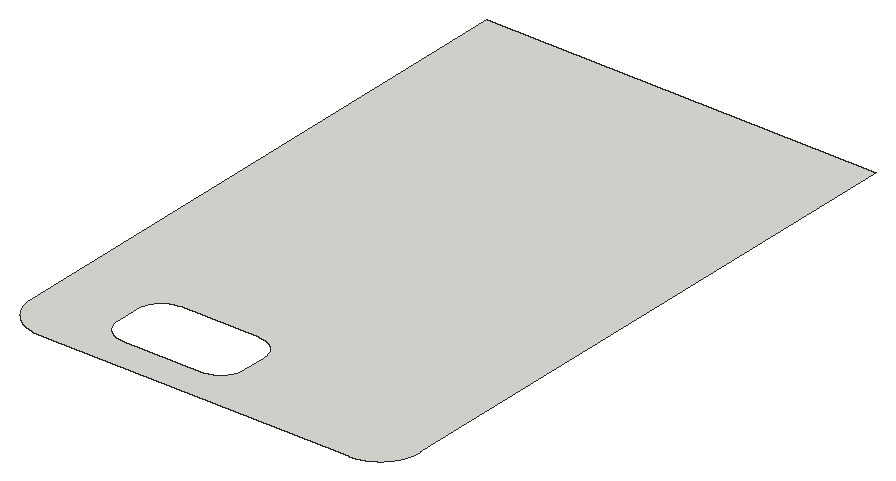
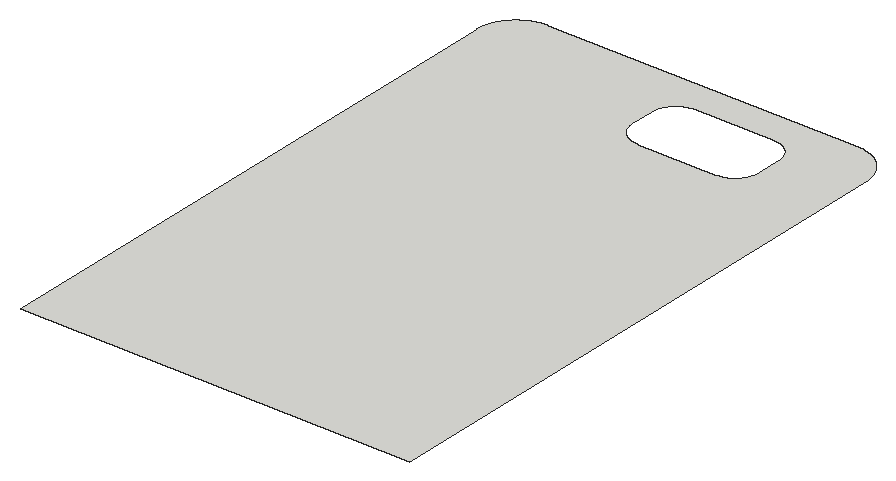
# SketchUp Ruby script. Lengths in inches.
U = 1.inch
M = Sketchup.active_model
def pt(a) = Geom::Point3d.new(a.map { |v| v * U })
def face(e, loops, mat)
  f = e.add_face(loops[0].map { |a| pt(a) })
  loops[1..].each { |l| e.add_face(l.map { |a| pt(a) }).erase! }
  f.material = f.back_material = mat if mat
  f
end
# faces: each face lists its corners as indices into pts; further lists are holes
def faces(e, pts, list, mat = nil) = list.each { |f| face(e, (f[0].is_a?(Array) ? f : [f]).map { |l| l.map { |i| pts[i] } }, mat) }
# xy, xz, yz: faces in a plane at the given z, y or x. An outline is a flat list of corners, or four numbers for a rectangle; further outlines are holes
def ring(l) = l.size == 4 ? [[l[0], l[1]], [l[2], l[1]], [l[2], l[3]], [l[0], l[3]]] : l.each_slice(2).to_a
def flat(e, list, mat, &to3) = list.each { |f| face(e, (f[0].is_a?(Array) ? f : [f]).map { |l| ring(l).map { |u, v| to3.(u, v) } }, mat) }
def xy(e, z, list, mat = nil) = flat(e, list, mat) { |x, y| [x, y, z] }
def xz(e, y, list, mat = nil) = flat(e, list, mat) { |x, z| [x, y, z] }
def yz(e, x, list, mat = nil) = flat(e, list, mat) { |y, z| [x, y, z] }
def lines(e, pts, list) = list.each { |a, b| e.add_line(pt(pts[a]), pt(pts[b])) }
# prism: a flat outline (further loops are holes) pulled along v
def prism(e, loops, v, mat = nil)
  f = face(e, loops, mat); d = Geom::Vector3d.new(v.map { |x| x * U })
  f.pushpull(f.normal.samedirection?(d) ? d.length : -d.length)
end
def box(e, o, s, mat = nil) = prism(e, [[o, [o[0] + s[0], o[1], o[2]], [o[0] + s[0], o[1] + s[1], o[2]], [o[0], o[1] + s[1], o[2]]]], [0, 0, s[2]], mat)
def at(x, y, z, deg = 0) = Geom::Transformation.translation(pt([x, y, z])) * Geom::Transformation.rotation(ORIGIN, Z_AXIS, deg.degrees)
def axes(o, x, y, z) = Geom::Transformation.new([*x, 0, *y, 0, *z, 0, *pt(o).to_a, 1])
def part(name) = M.definitions.add(name)
# library, detail: a bought-in or finely detailed component or shape, given as its bounding box
def library(name, o, s) = part(name).tap { |d| box(d.entities, o, s) }
def detail(e, o, s) = box(e.add_group.entities, o, s)
def put(e, d, t, mat = nil) = e.add_instance(d, t).tap { |i| i.material = mat if mat }
def group(e, t, mat = nil) = e.add_group.tap { |g| g.transformation = t; g.material = mat if mat }.entities
root = M.entities
xy(root,357,[[[38.61,204,270.39,204,270.79,204.01,271.18,204.02,271.57,204.04,271.96,204.0625,272.35,204.09,272.75,204.125,273.14,204.16,273.92,204.26,274.3,204.31,275.08,204.43,275.47,204.5,275.85,204.58,276.24,204.66,276.62,204.74,277.38,204.92,277.76,205.02,278.14,205.125,278.52,205.24,278.9,205.35,279.64,205.59,280.38,205.85,280.75,205.99,281.12,206.14,281.48,206.28,281.84,206.4375,282.2,206.59,282.56,206.76,282.92,206.92,283.27,207.09,283.97,207.45,284.31,207.64,284.66,207.83,285,208.02,285.34,208.22,285.67,208.42,286.01,208.63,286.34,208.84,286.67,209.06,286.99,209.28,287.3125,209.5,287.63,209.73,287.95,209.96,288.57,210.44,288.88,210.6875,289.18,210.93,289.48,211.1875,289.78,211.44,290.07,211.71,290.36,211.97,290.65,212.24,290.93,212.51,291.49,213.07,291.76,213.35,292.03,213.64,292.29,213.93,292.56,214.22,292.8125,214.52,293.07,214.82,293.3125,215.12,293.56,215.43,294.04,216.05,294.27,216.37,294.5,216.6875,294.72,217.01,294.94,217.33,295.16,217.66,295.37,217.99,295.58,218.33,295.78,218.66,295.98,219,296.17,219.34,296.36,219.69,296.55,220.03,296.91,220.73,297.08,221.08,297.24,221.44,297.41,221.8,297.5625,222.16,297.72,222.52,297.86,222.88,298.01,223.25,298.15,223.62,298.41,224.36,298.65,225.1,298.76,225.48,298.875,225.86,298.98,226.24,299.08,226.62,299.26,227.38,299.34,227.76,299.42,228.15,299.5,228.53,299.57,228.92,299.69,229.7,299.74,230.08,299.84,230.86,299.875,231.25,299.91,231.65,299.9375,232.04,299.96,232.43,299.98,232.82,299.99,233.21,300,233.61,300,660,9,660,9,233.61,9.01,233.21,9.02,232.82,9.04,232.43,9.0625,232.04,9.09,231.65,9.125,231.25,9.16,230.86,9.26,230.08,9.31,229.7,9.43,228.92,9.5,228.53,9.58,228.15,9.66,227.76,9.74,227.38,9.92,226.62,10.02,226.24,10.125,225.86,10.24,225.48,10.35,225.1,10.59,224.36,10.85,223.62,10.99,223.25,11.14,222.88,11.28,222.52,11.4375,222.16,11.59,221.8,11.76,221.44,11.92,221.08,12.09,220.73,12.45,220.03,12.64,219.69,12.83,219.34,13.02,219,13.22,218.66,13.42,218.33,13.63,217.99,13.84,217.66,14.06,217.33,14.28,217.01,14.5,216.6875,14.73,216.37,14.96,216.05,15.44,215.43,15.6875,215.12,15.93,214.82,16.1875,214.52,16.44,214.22,16.71,213.93,16.97,213.64,17.24,213.35,17.51,213.07,18.07,212.51,18.35,212.24,18.64,211.97,18.93,211.71,19.22,211.44,19.52,211.1875,19.82,210.93,20.12,210.6875,20.43,210.44,21.05,209.96,21.37,209.73,21.6875,209.5,22.01,209.28,22.33,209.06,22.66,208.84,22.99,208.63,23.33,208.42,23.66,208.22,24,208.02,24.34,207.83,24.69,207.64,25.03,207.45,25.73,207.09,26.08,206.92,26.44,206.76,26.8,206.59,27.16,206.4375,27.52,206.28,27.88,206.14,28.25,205.99,28.62,205.85,29.36,205.59,30.1,205.35,30.48,205.24,30.86,205.125,31.24,205.02,31.62,204.92,32.38,204.74,32.76,204.66,33.15,204.58,33.53,204.5,33.92,204.43,34.7,204.31,35.08,204.26,35.86,204.16,36.25,204.125,36.65,204.09,37.04,204.0625,37.43,204.04,37.82,204.02,38.21,204.01],[82,228,81.43,228.01,80.87,228.04,80.31,228.08,79.74,228.14,79.18,228.22,78.63,228.32,78.07,228.43,77.52,228.57,76.98,228.71,76.4375,228.88,75.9,229.0625,75.375,229.26,74.85,229.48,74.34,229.71,73.83,229.96,73.33,230.23,72.84,230.51,72.36,230.8,71.88,231.11,71.42,231.4375,70.97,231.78,70.53,232.13,70.1,232.5,69.68,232.88,69.27,233.27,68.88,233.68,68.5,234.1,68.13,234.53,67.78,234.97,67.4375,235.42,67.11,235.88,66.8,236.36,66.51,236.84,66.23,237.33,65.96,237.83,65.71,238.34,65.48,238.85,65.26,239.375,65.0625,239.9,64.88,240.4375,64.71,240.98,64.57,241.52,64.43,242.07,64.32,242.63,64.22,243.18,64.14,243.74,64.08,244.31,64.04,244.87,64.01,245.43,64,246,64,264,64.01,264.57,64.04,265.13,64.08,265.69,64.14,266.26,64.22,266.82,64.32,267.37,64.43,267.93,64.57,268.48,64.71,269.02,64.88,269.5625,65.0625,270.1,65.26,270.625,65.48,271.15,65.71,271.66,65.96,272.17,66.23,272.67,66.51,273.16,66.8,273.64,67.11,274.12,67.4375,274.58,67.78,275.03,68.13,275.47,68.5,275.9,68.88,276.32,69.27,276.73,69.68,277.12,70.1,277.5,70.53,277.87,70.97,278.22,71.42,278.5625,71.88,278.89,72.36,279.2,72.84,279.49,73.33,279.77,73.83,280.04,74.34,280.29,74.85,280.52,75.375,280.74,75.9,280.9375,76.4375,281.12,76.98,281.29,77.52,281.43,78.07,281.57,78.63,281.68,79.18,281.78,79.74,281.86,80.31,281.92,80.87,281.96,81.43,281.99,82,282,141,282,141.57,281.99,142.13,281.96,142.69,281.92,143.26,281.86,143.82,281.78,144.37,281.68,144.93,281.57,145.48,281.43,146.02,281.29,146.5625,281.12,147.1,280.9375,147.625,280.74,148.15,280.52,148.66,280.29,149.17,280.04,149.67,279.77,150.16,279.49,150.64,279.2,151.12,278.89,151.58,278.5625,152.03,278.22,152.47,277.87,152.9,277.5,153.32,277.12,153.73,276.73,154.12,276.32,154.5,275.9,154.87,275.47,155.22,275.03,155.5625,274.58,155.89,274.12,156.2,273.64,156.49,273.16,156.77,272.67,157.04,272.17,157.29,271.66,157.52,271.15,157.74,270.625,157.9375,270.1,158.12,269.5625,158.29,269.02,158.43,268.48,158.57,267.93,158.68,267.37,158.78,266.82,158.86,266.26,158.92,265.69,158.96,265.13,158.99,264.57,159,264,159,246,158.99,245.43,158.96,244.87,158.92,244.31,158.86,243.74,158.78,243.18,158.68,242.63,158.57,242.07,158.43,241.52,158.29,240.98,158.12,240.4375,157.9375,239.9,157.74,239.375,157.52,238.85,157.29,238.34,157.04,237.83,156.77,237.33,156.49,236.84,156.2,236.36,155.89,235.88,155.5625,235.42,155.22,234.97,154.87,234.53,154.5,234.1,154.12,233.68,153.73,233.27,153.32,232.88,152.9,232.5,152.47,232.13,152.03,231.78,151.58,231.4375,151.12,231.11,150.64,230.8,150.16,230.51,149.67,230.23,149.17,229.96,148.66,229.71,148.15,229.48,147.625,229.26,147.1,229.0625,146.5625,228.88,146.02,228.71,145.48,228.57,144.93,228.43,144.37,228.32,143.82,228.22,143.26,228.14,142.69,228.08,142.13,228.04,141.57,228.01,141,228]]])
